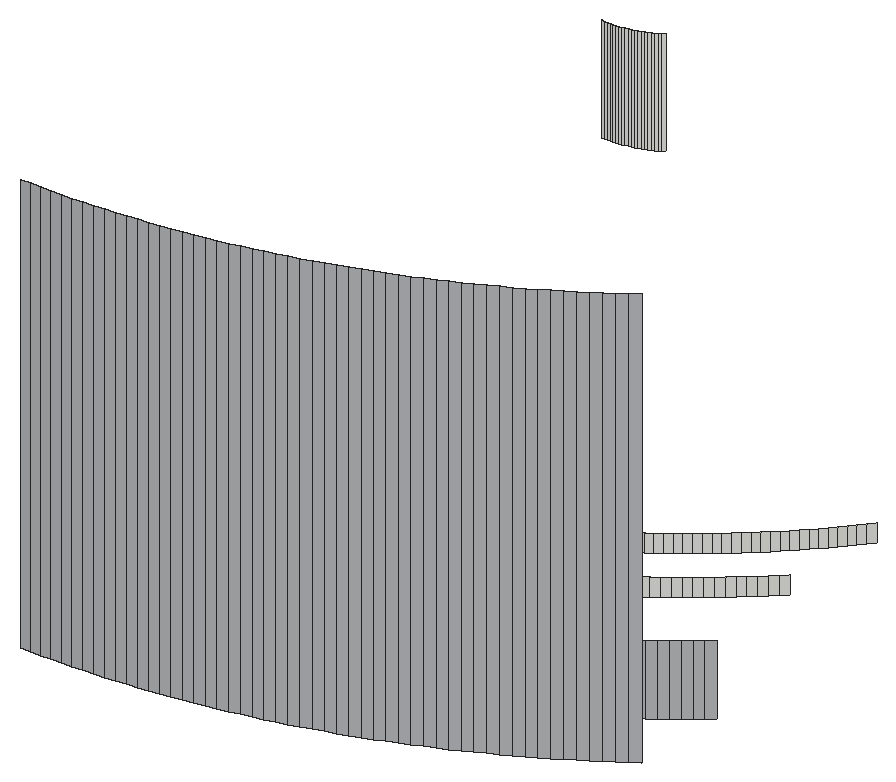
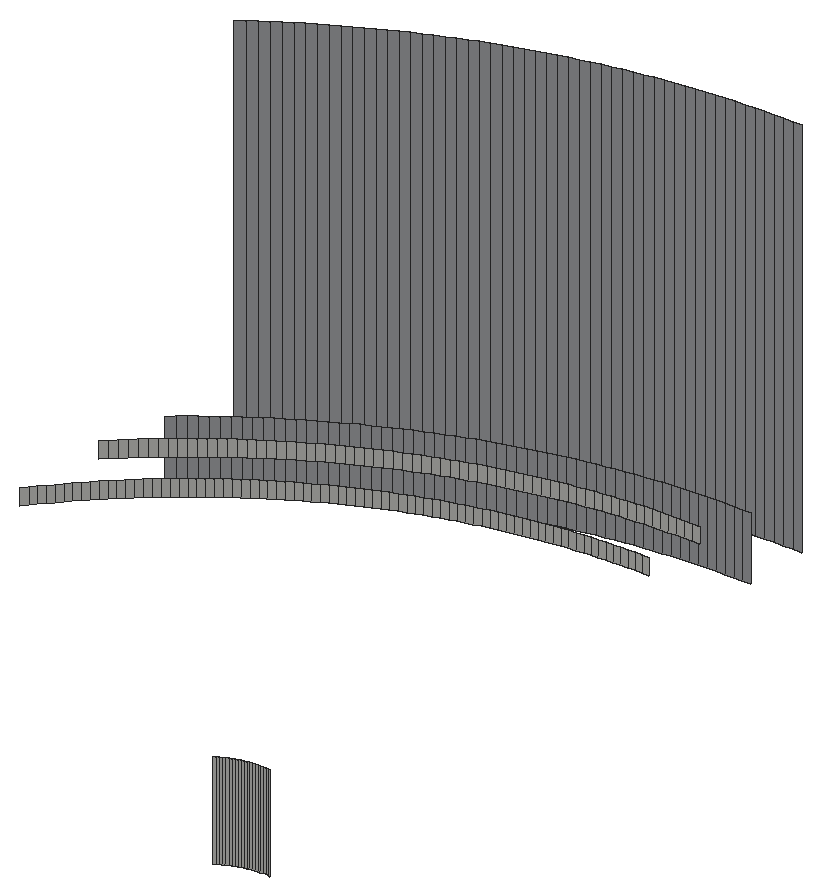
# SketchUp Ruby script. Lengths in inches.
U = 1.inch
M = Sketchup.active_model
def pt(a) = Geom::Point3d.new(a.map { |v| v * U })
def face(e, loops, mat)
  f = e.add_face(loops[0].map { |a| pt(a) })
  loops[1..].each { |l| e.add_face(l.map { |a| pt(a) }).erase! }
  f.material = f.back_material = mat if mat
  f
end
# faces: each face lists its corners as indices into pts; further lists are holes
def faces(e, pts, list, mat = nil) = list.each { |f| face(e, (f[0].is_a?(Array) ? f : [f]).map { |l| l.map { |i| pts[i] } }, mat) }
# xy, xz, yz: faces in a plane at the given z, y or x. An outline is a flat list of corners, or four numbers for a rectangle; further outlines are holes
def ring(l) = l.size == 4 ? [[l[0], l[1]], [l[2], l[1]], [l[2], l[3]], [l[0], l[3]]] : l.each_slice(2).to_a
def flat(e, list, mat, &to3) = list.each { |f| face(e, (f[0].is_a?(Array) ? f : [f]).map { |l| ring(l).map { |u, v| to3.(u, v) } }, mat) }
def xy(e, z, list, mat = nil) = flat(e, list, mat) { |x, y| [x, y, z] }
def xz(e, y, list, mat = nil) = flat(e, list, mat) { |x, z| [x, y, z] }
def yz(e, x, list, mat = nil) = flat(e, list, mat) { |y, z| [x, y, z] }
def lines(e, pts, list) = list.each { |a, b| e.add_line(pt(pts[a]), pt(pts[b])) }
# prism: a flat outline (further loops are holes) pulled along v
def prism(e, loops, v, mat = nil)
  f = face(e, loops, mat); d = Geom::Vector3d.new(v.map { |x| x * U })
  f.pushpull(f.normal.samedirection?(d) ? d.length : -d.length)
end
def box(e, o, s, mat = nil) = prism(e, [[o, [o[0] + s[0], o[1], o[2]], [o[0] + s[0], o[1] + s[1], o[2]], [o[0], o[1] + s[1], o[2]]]], [0, 0, s[2]], mat)
def at(x, y, z, deg = 0) = Geom::Transformation.translation(pt([x, y, z])) * Geom::Transformation.rotation(ORIGIN, Z_AXIS, deg.degrees)
def axes(o, x, y, z) = Geom::Transformation.new([*x, 0, *y, 0, *z, 0, *pt(o).to_a, 1])
def part(name) = M.definitions.add(name)
# library, detail: a bought-in or finely detailed component or shape, given as its bounding box
def library(name, o, s) = part(name).tap { |d| box(d.entities, o, s) }
def detail(e, o, s) = box(e.add_group.entities, o, s)
def put(e, d, t, mat = nil) = e.add_instance(d, t).tap { |i| i.material = mat if mat }
def group(e, t, mat = nil) = e.add_group.tap { |g| g.transformation = t; g.material = mat if mat }.entities
root = M.entities
M.materials.add("1427 AP 686 ARMOUR-N").color = [184, 186, 189]
p = [[141.288,129.926,252],[140.998,129.924,252],[140.998,129.924,240],[141.003,129.924,240],[141.288,129.926,240],[141.578,129.931,252],
  [141.578,129.931,240],[141.868,129.94,252],[141.868,129.94,240],[142.158,129.952,252],[142.158,129.952,240],[142.447,129.968,252],
  [142.447,129.968,240],[142.737,129.987,252],[142.737,129.987,240],[143.026,130.01,252],[143.026,130.01,240],[143.315,130.036,252],
  [143.315,130.036,240],[143.603,130.066,252],[143.603,130.066,240],[143.891,130.099,252],[143.891,130.099,240],[144.179,130.136,252],
  [144.179,130.136,240],[144.466,130.176,252],[144.466,130.176,240],[144.753,130.22,252],[144.753,130.22,240],[145.039,130.267,252],
  [145.039,130.267,240],[145.325,130.318,252],[145.325,130.318,240],[145.61,130.372,252],[145.61,130.372,240],[145.894,130.429,252],
  [145.894,130.429,240],[146.177,130.49,252],[146.177,130.49,240],[146.46,130.554,252],[146.46,130.554,240],[146.742,130.622,252],
  [146.742,130.622,240],[147.023,130.693,252],[147.023,130.693,240],[147.304,130.767,252],[147.304,130.767,240],[147.583,130.845,252],
  [147.583,130.845,240],[147.861,130.926,252],[147.861,130.926,240],[148.139,131.011,252],[148.139,131.011,240],[148.415,131.099,252],
  [148.415,131.099,240],[148.69,131.19,252],[148.69,131.19,240],[148.964,131.285,252],[148.964,131.285,240],[149.237,131.383,252],
  [149.237,131.383,240],[149.509,131.484,252],[149.509,131.484,240],[149.78,131.588,252],[149.78,131.588,240],[150.049,131.696,252],
  [150.049,131.696,240],[150.317,131.807,252],[150.317,131.807,240],[150.583,131.921,252],[150.583,131.921,240],[141.264,131.926,240],
  [140.992,131.924,240],[140.992,131.924,242],[141.264,131.926,242],[141.53,131.931,240],[141.53,131.931,242],[141.796,131.939,240],
  [141.796,131.939,242],[142.061,131.95,240],[142.061,131.95,242],[150.849,132.039,252],[150.849,132.039,240],[142.327,131.965,240],
  [142.327,131.965,242],[142.592,131.982,240],[142.592,131.982,242],[142.857,132.003,240],[142.857,132.003,242],[143.122,132.027,240],
  [143.122,132.027,242],[143.386,132.054,240],[143.386,132.054,242],[151.112,132.159,252],[151.112,132.159,240],[143.65,132.085,240],
  [143.65,132.085,242],[143.914,132.118,240],[143.914,132.118,242],[144.177,132.155,240],[144.177,132.155,242],[144.44,132.195,240],
  [144.44,132.195,242],[144.702,132.238,240],[144.702,132.238,242],[144.964,132.285,240],[144.964,132.285,242],[151.375,132.283,252],
  [151.375,132.283,240],[145.225,132.334,240],[145.225,132.334,242],[145.486,132.387,240],[145.486,132.387,242],[151.635,132.41,252],
  [151.635,132.41,240],[145.746,132.443,240],[145.746,132.443,242],[146.005,132.502,240],[146.005,132.502,242],[151.894,132.54,252],
  [151.894,132.54,240],[146.263,132.564,240],[146.263,132.564,242],[152.152,132.673,252],[152.152,132.673,240],[146.521,132.629,240],
  [146.521,132.629,242],[146.778,132.697,240],[146.778,132.697,242],[147.034,132.769,240],[147.034,132.769,242],[152.408,132.81,252],
  [152.408,132.81,240],[147.289,132.843,240],[147.289,132.843,242],[147.544,132.921,240],[147.544,132.921,242],[152.662,132.949,252],
  [152.662,132.949,240],[147.797,133.001,240],[147.797,133.001,242],[152.915,133.092,252],[152.915,133.092,240],[148.049,133.085,240],
  [148.049,133.085,242],[148.301,133.172,240],[148.301,133.172,242],[153.166,133.237,252],[153.166,133.237,240],[148.551,133.261,240],
  [148.551,133.261,242],[153.415,133.386,252],[153.415,133.386,240],[148.8,133.354,240],[148.8,133.354,242],[149.048,133.45,240],
  [149.048,133.45,242],[149.295,133.549,240],[149.295,133.549,242],[153.662,133.537,252],[153.662,133.537,240],[149.54,133.65,240],
  [149.54,133.65,242],[153.908,133.692,252],[153.908,133.692,240],[149.785,133.755,240],[149.785,133.755,242],[154.151,133.849,252],
  [154.151,133.849,240],[150.028,133.863,240],[150.028,133.863,242],[154.393,134.009,252],[154.393,134.009,240],[150.269,133.973,240],
  [150.269,133.973,242],[150.51,134.087,240],[150.51,134.087,242],[154.632,134.173,252],[154.632,134.173,240],[150.749,134.203,240],
  [150.749,134.203,242],[150.986,134.322,240],[150.986,134.322,242],[154.87,134.339,252],[154.87,134.339,240],[151.223,134.444,240],
  [151.223,134.444,242],[155.106,134.508,252],[155.106,134.508,240],[151.457,134.569,240],[151.457,134.569,242],[151.69,134.697,240],
  [151.69,134.697,242],[151.922,134.828,240],[151.922,134.828,242],[152.152,134.961,240],[152.152,134.961,242],[152.38,135.097,240],
  [152.38,135.097,242],[152.607,135.236,240],[152.607,135.236,242],[152.832,135.378,240],[152.832,135.378,242],[153.055,135.522,240],
  [153.055,135.522,242],[153.277,135.669,240],[153.277,135.669,242],[153.496,135.819,240],[153.496,135.819,242],[153.714,135.971,240],
  [153.714,135.971,242],[153.93,136.126,240],[153.93,136.126,242],[154.144,136.284,240],[154.144,136.284,242],[154.356,136.444,240],
  [154.356,136.444,242],[154.567,136.606,240],[154.567,136.606,242],[154.775,136.772,240],[154.775,136.772,242],[154.981,136.939,240],
  [154.981,136.939,242],[155.185,137.109,240],[155.185,137.109,242],[141.24,133.926,242],[140.986,133.924,242],[140.986,133.924,242.5],
  [141.24,133.926,242.5],[141.482,133.93,242],[141.482,133.93,242.5],[141.723,133.9375,242],[141.723,133.9375,242.5],[141.965,133.948,242],
  [141.965,133.948,242.5],[142.206,133.961,242],[142.206,133.961,242.5],[142.447,133.977,242],[142.447,133.977,242.5],[142.688,133.996,242],
  [142.688,133.996,242.5],[142.929,134.018,242],[142.929,134.018,242.5],[143.169,134.043,242],[143.169,134.043,242.5],[143.409,134.07,242],
  [143.409,134.07,242.5],[143.649,134.101,242],[143.649,134.101,242.5],[143.888,134.134,242],[143.888,134.134,242.5],[144.127,134.171,242],
  [144.127,134.171,242.5],[144.366,134.21,242],[144.366,134.21,242.5],[144.604,134.252,242],[144.604,134.252,242.5],[144.841,134.297,242],
  [144.841,134.297,242.5],[145.078,134.345,242],[145.078,134.345,242.5],[145.314,134.396,242],[145.314,134.396,242.5],[145.55,134.449,242],
  [145.55,134.449,242.5],[145.785,134.506,242],[145.785,134.506,242.5],[146.019,134.565,242],[146.019,134.565,242.5],[146.253,134.627,242],
  [146.253,134.627,242.5],[146.485,134.692,242],[146.485,134.692,242.5],[146.717,134.76,242],[146.717,134.76,242.5],[146.949,134.83,242],
  [146.949,134.83,242.5],[147.179,134.903,242],[147.179,134.903,242.5],[147.408,134.979,242],[147.408,134.979,242.5],[147.637,135.058,242],
  [147.637,135.058,242.5],[147.864,135.14,242],[147.864,135.14,242.5],[148.091,135.224,242],[148.091,135.224,242.5],[148.316,135.311,242],
  [148.316,135.311,242.5],[148.541,135.401,242],[148.541,135.401,242.5],[148.764,135.493,242],[148.764,135.493,242.5],[148.986,135.589,242],
  [148.986,135.589,242.5],[149.207,135.686,242],[149.207,135.686,242.5],[149.427,135.787,242],[149.427,135.787,242.5],[149.645,135.89,242],
  [149.645,135.89,242.5],[140.98,135.924,242],[141.216,135.926,242],[141.216,135.926,242.5],[140.98,135.924,242.5],[141.433,135.93,242],
  [141.433,135.93,242.5],[141.651,135.936,242],[141.651,135.936,242.5],[141.868,135.946,242],[141.868,135.946,242.5],[142.085,135.957,242],
  [142.085,135.957,242.5],[149.863,135.996,242],[149.863,135.996,242.5],[142.302,135.972,242],[142.302,135.972,242.5],[142.519,135.989,242],
  [142.519,135.989,242.5],[142.736,136.009,242],[142.736,136.009,242.5],[142.952,136.031,242],[142.952,136.031,242.5],[143.168,136.056,242],
  [143.168,136.056,242.5],[150.079,136.104,242],[150.079,136.104,242.5],[143.384,136.083,242],[143.384,136.083,242.5],[143.599,136.113,242],
  [143.599,136.113,242.5],[143.814,136.146,242],[143.814,136.146,242.5],[144.029,136.181,242],[144.029,136.181,242.5],[150.293,136.215,242],
  [150.293,136.215,242.5],[144.243,136.219,242],[144.243,136.219,242.5],[144.457,136.26,242],[144.457,136.26,242.5],[150.506,136.329,242],
  [150.506,136.329,242.5],[144.67,136.303,242],[144.67,136.303,242.5],[144.883,136.349,242],[144.883,136.349,242.5],[145.095,136.397,242],
  [145.095,136.397,242.5],[150.718,136.445,242],[150.718,136.445,242.5],[145.306,136.448,242],[145.306,136.448,242.5],[145.517,136.501,242],
  [145.517,136.501,242.5],[150.929,136.564,242],[150.929,136.564,242.5],[145.727,136.557,242],[145.727,136.557,242.5],[145.937,136.615,242],
  [145.937,136.615,242.5],[146.146,136.676,242],[146.146,136.676,242.5],[151.138,136.685,242],[151.138,136.685,242.5],[146.354,136.74,242],
  [146.354,136.74,242.5],[146.561,136.805,242],[146.561,136.805,242.5],[151.346,136.809,242],[151.346,136.809,242.5],[146.767,136.874,242],
  [146.767,136.874,242.5],[151.552,136.935,242],[151.552,136.935,242.5],[146.973,136.945,242],[146.973,136.945,242.5],[147.178,137.018,242],
  [147.178,137.018,242.5],[151.756,137.064,242],[151.756,137.064,242.5],[147.382,137.094,242],[147.382,137.094,242.5],[147.584,137.173,242],
  [147.584,137.173,242.5],[151.959,137.195,242],[151.959,137.195,242.5],[147.786,137.253,242],[147.786,137.253,242.5],[152.16,137.329,242],
  [152.16,137.329,242.5],[147.987,137.337,242],[147.987,137.337,242.5],[148.187,137.422,242],[148.187,137.422,242.5],[152.36,137.465,242],
  [152.36,137.465,242.5],[148.386,137.51,242],[148.386,137.51,242.5],[148.584,137.601,242],[148.584,137.601,242.5],[152.558,137.603,242],
  [152.558,137.603,242.5],[148.781,137.694,242],[148.781,137.694,242.5],[152.755,137.744,242],[152.755,137.744,242.5],[148.976,137.789,242],
  [148.976,137.789,242.5],[152.949,137.887,242],[152.949,137.887,242.5],[149.171,137.886,242],[149.171,137.886,242.5],[149.364,137.986,242],
  [149.364,137.986,242.5],[153.142,138.033,242],[153.142,138.033,242.5],[149.556,138.089,242],[149.556,138.089,242.5],[153.333,138.181,242],
  [153.333,138.181,242.5],[149.746,138.193,242],[149.746,138.193,242.5],[149.936,138.3,242],[149.936,138.3,242.5],[153.523,138.331,242],
  [153.523,138.331,242.5],[150.124,138.409,242],[150.124,138.409,242.5],[153.71,138.483,242],[153.71,138.483,242.5],[150.311,138.52,242],
  [150.311,138.52,242.5],[150.496,138.634,242],[150.496,138.634,242.5],[153.896,138.638,242],[153.896,138.638,242.5],[150.68,138.75,242],
  [150.68,138.75,242.5],[154.08,138.795,242],[154.08,138.795,242.5],[150.863,138.868,242],[150.863,138.868,242.5],[154.261,138.954,242],
  [154.261,138.954,242.5],[151.044,138.988,242],[151.044,138.988,242.5],[151.224,139.111,242],[151.224,139.111,242.5],[154.441,139.116,242],
  [154.441,139.116,242.5],[151.402,139.235,242],[151.402,139.235,242.5],[154.619,139.279,242],[154.619,139.279,242.5],[151.579,139.362,242],
  [151.579,139.362,242.5],[154.795,139.445,242],[154.795,139.445,242.5],[151.754,139.491,242],[151.754,139.491,242.5],[154.969,139.612,242],
  [154.969,139.612,242.5],[151.928,139.622,242],[151.928,139.622,242.5],[152.1,139.755,242],[152.1,139.755,242.5],[155.141,139.782,242],
  [155.141,139.782,242.5],[152.27,139.89,242],[152.27,139.89,242.5],[152.439,140.028,242],[152.439,140.028,242.5],[152.606,140.167,242],
  [152.606,140.167,242.5],[152.771,140.308,242],[152.771,140.308,242.5],[152.935,140.451,242],[152.935,140.451,242.5],[153.097,140.597,242],
  [153.097,140.597,242.5],[153.257,140.744,242],[153.257,140.744,242.5],[153.416,140.893,242],[153.416,140.893,242.5],[153.572,141.044,242],
  [153.572,141.044,242.5],[153.727,141.197,242],[153.727,141.197,242.5],[153.88,141.351,242],[153.88,141.351,242.5],[154.031,141.508,242],
  [154.031,141.508,242.5],[154.18,141.666,242],[154.18,141.666,242.5],[154.327,141.826,242],[154.327,141.826,242.5],[154.472,141.988,242],
  [154.472,141.988,242.5],[154.616,142.152,242],[154.616,142.152,242.5],[154.757,142.317,242],[154.757,142.317,242.5],[154.896,142.484,242],
  [154.896,142.484,242.5],[155.033,142.653,242],[155.033,142.653,242.5],[155.168,142.824,242],[155.168,142.824,242.5],[138.921,153.426,242],
  [138.843,153.429,242],[138.843,153.429,245],[138.921,153.426,245],[139,153.424,242],[139,153.424,245],[139.079,153.426,242],
  [139.079,153.426,245],[139.157,153.429,242],[139.157,153.429,245],[139.235,153.435,242],[139.235,153.435,245],[139.313,153.444,242],
  [139.313,153.444,245],[139.391,153.455,242],[139.391,153.455,245],[139.468,153.469,242],[139.468,153.469,245],[139.545,153.485,242],
  [139.545,153.485,245],[139.622,153.503,242],[139.622,153.503,245],[139.697,153.524,242],[139.697,153.524,245],[139.773,153.547,242],
  [139.773,153.547,245],[139.847,153.572,242],[139.847,153.572,245],[139.92,153.6,242],[139.92,153.6,245],[139.993,153.63,242],
  [139.993,153.63,245],[140.064,153.662,242],[140.064,153.662,245],[140.135,153.697,242],[140.135,153.697,245],[140.204,153.734,242],
  [140.204,153.734,245],[140.273,153.773,242],[140.273,153.773,245],[140.34,153.814,242],[140.34,153.814,245]]
faces(root,p,[[0,1,2,3,4],[5,0,4,6],[7,5,6,8],[9,7,8,10],[11,9,10,12],[13,11,12,14],[15,13,14,16],[17,15,16,18],
  [19,17,18,20],[21,19,20,22],[23,21,22,24],[25,23,24,26],[27,25,26,28],[29,27,28,30],[31,29,30,32],[33,31,32,34],
  [35,33,34,36],[37,35,36,38],[39,37,38,40],[41,39,40,42],[43,41,42,44],[45,43,44,46],[47,45,46,48],[49,47,48,50],
  [51,49,50,52],[53,51,52,54],[55,53,54,56],[57,55,56,58],[59,57,58,60],[61,59,60,62],[63,61,62,64],[65,63,64,66],
  [67,65,66,68],[69,67,68,70],[71,72,73,74],[75,71,74,76],[77,75,76,78],[79,77,78,80],[81,69,70,82],[83,79,80,84],
  [85,83,84,86],[87,85,86,88],[89,87,88,90],[91,89,90,92],[93,81,82,94],[95,91,92,96],[97,95,96,98],[99,97,98,100],
  [101,99,100,102],[103,101,102,104],[105,103,104,106],[107,93,94,108],[109,105,106,110],[111,109,110,112],[113,107,108,114],[115,111,112,116],
  [117,115,116,118],[119,113,114,120],[121,117,118,122],[123,119,120,124],[125,121,122,126],[127,125,126,128],[129,127,128,130],[131,123,124,132],
  [133,129,130,134],[135,133,134,136],[137,131,132,138],[139,135,136,140],[141,137,138,142],[143,139,140,144],[145,143,144,146],[147,141,142,148],
  [149,145,146,150],[151,147,148,152],[153,149,150,154],[155,153,154,156],[157,155,156,158],[159,151,152,160],[161,157,158,162],[163,159,160,164],
  [165,161,162,166],[167,163,164,168],[169,165,166,170],[171,167,168,172],[173,169,170,174],[175,173,174,176],[177,171,172,178],[179,175,176,180],
  [181,179,180,182],[183,177,178,184],[185,181,182,186],[187,183,184,188],[189,185,186,190],[191,189,190,192],[193,191,192,194],[195,193,194,196],
  [197,195,196,198],[199,197,198,200],[201,199,200,202],[203,201,202,204],[205,203,204,206],[207,205,206,208],[209,207,208,210],[211,209,210,212],
  [213,211,212,214],[215,213,214,216],[217,215,216,218],[219,217,218,220],[221,219,220,222],[223,221,222,224]],"1427 AP 686 ARMOUR-N")
faces(root,p,[[225,226,227,228],[229,225,228,230],[231,229,230,232],[233,231,232,234],[235,233,234,236],[237,235,236,238],[239,237,238,240],[241,239,240,242],
  [243,241,242,244],[245,243,244,246],[247,245,246,248],[249,247,248,250],[251,249,250,252],[253,251,252,254],[255,253,254,256],[257,255,256,258],
  [259,257,258,260],[261,259,260,262],[263,261,262,264],[265,263,264,266],[267,265,266,268],[269,267,268,270],[271,269,270,272],[273,271,272,274],
  [275,273,274,276],[277,275,276,278],[279,277,278,280],[281,279,280,282],[283,281,282,284],[285,283,284,286],[287,285,286,288],[289,287,288,290],
  [291,289,290,292],[293,291,292,294],[295,293,294,296],[297,295,296,298],[299,297,298,300],[301,302,303,304],[302,305,306,303],[305,307,308,306],
  [307,309,310,308],[309,311,312,310],[313,299,300,314],[311,315,316,312],[315,317,318,316],[317,319,320,318],[319,321,322,320],[321,323,324,322],
  [325,313,314,326],[323,327,328,324],[327,329,330,328],[329,331,332,330],[331,333,334,332],[335,325,326,336],[333,337,338,334],[337,339,340,338],
  [341,335,336,342],[339,343,344,340],[343,345,346,344],[345,347,348,346],[349,341,342,350],[347,351,352,348],[351,353,354,352],[355,349,350,356],
  [353,357,358,354],[357,359,360,358],[359,361,362,360],[363,355,356,364],[361,365,366,362],[365,367,368,366],[369,363,364,370],[367,371,372,368],
  [373,369,370,374],[371,375,376,372],[375,377,378,376],[379,373,374,380],[377,381,382,378],[381,383,384,382],[385,379,380,386],[383,387,388,384],
  [389,385,386,390],[387,391,392,388],[391,393,394,392],[395,389,390,396],[393,397,398,394],[397,399,400,398],[401,395,396,402],[399,403,404,400],
  [405,401,402,406],[403,407,408,404],[409,405,406,410],[407,411,412,408],[411,413,414,412],[415,409,410,416],[413,417,418,414],[419,415,416,420],
  [417,421,422,418],[421,423,424,422],[425,419,420,426],[423,427,428,424],[429,425,426,430],[427,431,432,428],[431,433,434,432],[435,429,430,436],
  [433,437,438,434],[439,435,436,440],[437,441,442,438],[443,439,440,444],[441,445,446,442],[445,447,448,446],[449,443,444,450],[447,451,452,448],
  [453,449,450,454],[451,455,456,452],[457,453,454,458],[455,459,460,456],[461,457,458,462],[459,463,464,460],[463,465,466,464],[467,461,462,468],
  [465,469,470,466],[469,471,472,470],[471,473,474,472],[473,475,476,474],[475,477,478,476],[477,479,480,478],[479,481,482,480],[481,483,484,482],
  [483,485,486,484],[485,487,488,486],[487,489,490,488],[489,491,492,490],[491,493,494,492],[493,495,496,494],[495,497,498,496],[497,499,500,498],
  [499,501,502,500],[501,503,504,502],[503,505,506,504],[505,507,508,506],[509,510,511,512],[513,509,512,514],[515,513,514,516],[517,515,516,518],
  [519,517,518,520],[521,519,520,522],[523,521,522,524],[525,523,524,526],[527,525,526,528],[529,527,528,530],[531,529,530,532],[533,531,532,534],
  [535,533,534,536],[537,535,536,538],[539,537,538,540],[541,539,540,542],[543,541,542,544],[545,543,544,546],[547,545,546,548],[549,547,548,550]])
